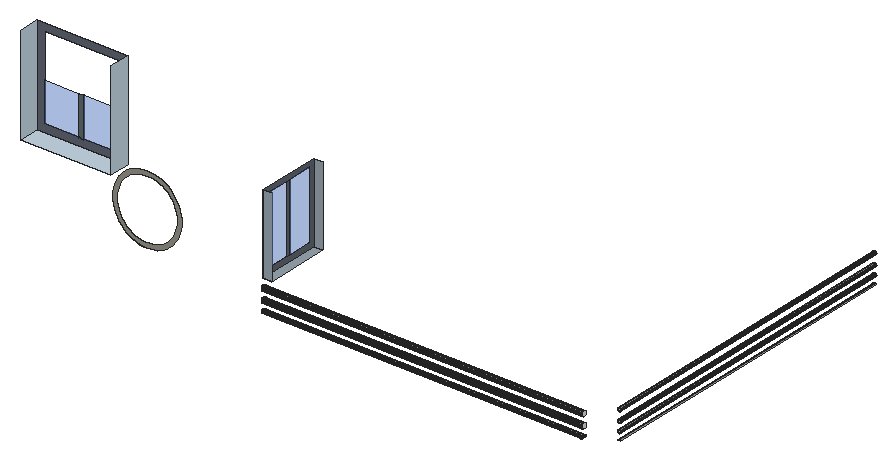
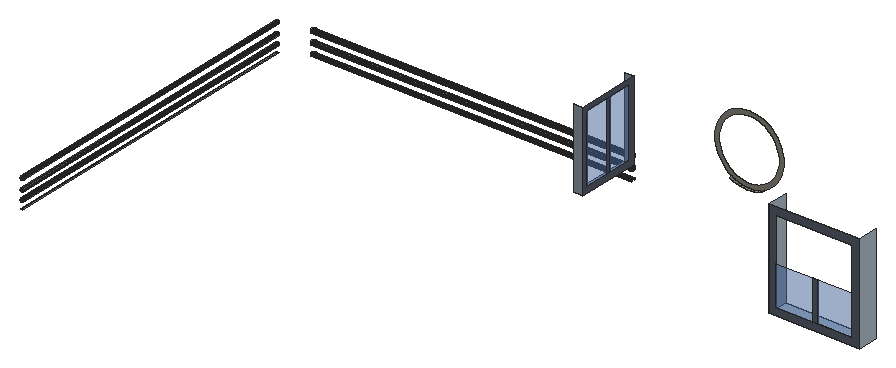
# SketchUp Ruby script. Lengths in inches.
U = 1.inch
M = Sketchup.active_model
def pt(a) = Geom::Point3d.new(a.map { |v| v * U })
def face(e, loops, mat)
  f = e.add_face(loops[0].map { |a| pt(a) })
  loops[1..].each { |l| e.add_face(l.map { |a| pt(a) }).erase! }
  f.material = f.back_material = mat if mat
  f
end
# faces: each face lists its corners as indices into pts; further lists are holes
def faces(e, pts, list, mat = nil) = list.each { |f| face(e, (f[0].is_a?(Array) ? f : [f]).map { |l| l.map { |i| pts[i] } }, mat) }
# xy, xz, yz: faces in a plane at the given z, y or x. An outline is a flat list of corners, or four numbers for a rectangle; further outlines are holes
def ring(l) = l.size == 4 ? [[l[0], l[1]], [l[2], l[1]], [l[2], l[3]], [l[0], l[3]]] : l.each_slice(2).to_a
def flat(e, list, mat, &to3) = list.each { |f| face(e, (f[0].is_a?(Array) ? f : [f]).map { |l| ring(l).map { |u, v| to3.(u, v) } }, mat) }
def xy(e, z, list, mat = nil) = flat(e, list, mat) { |x, y| [x, y, z] }
def xz(e, y, list, mat = nil) = flat(e, list, mat) { |x, z| [x, y, z] }
def yz(e, x, list, mat = nil) = flat(e, list, mat) { |y, z| [x, y, z] }
def lines(e, pts, list) = list.each { |a, b| e.add_line(pt(pts[a]), pt(pts[b])) }
# prism: a flat outline (further loops are holes) pulled along v
def prism(e, loops, v, mat = nil)
  f = face(e, loops, mat); d = Geom::Vector3d.new(v.map { |x| x * U })
  f.pushpull(f.normal.samedirection?(d) ? d.length : -d.length)
end
def box(e, o, s, mat = nil) = prism(e, [[o, [o[0] + s[0], o[1], o[2]], [o[0] + s[0], o[1] + s[1], o[2]], [o[0], o[1] + s[1], o[2]]]], [0, 0, s[2]], mat)
def at(x, y, z, deg = 0) = Geom::Transformation.translation(pt([x, y, z])) * Geom::Transformation.rotation(ORIGIN, Z_AXIS, deg.degrees)
def axes(o, x, y, z) = Geom::Transformation.new([*x, 0, *y, 0, *z, 0, *pt(o).to_a, 1])
def part(name) = M.definitions.add(name)
# library, detail: a bought-in or finely detailed component or shape, given as its bounding box
def library(name, o, s) = part(name).tap { |d| box(d.entities, o, s) }
def detail(e, o, s) = box(e.add_group.entities, o, s)
def put(e, d, t, mat = nil) = e.add_instance(d, t).tap { |i| i.material = mat if mat }
def group(e, t, mat = nil) = e.add_group.tap { |g| g.transformation = t; g.material = mat if mat }.entities
root = M.entities
M.materials.add("[Color M04]").color = [142, 142, 142]
M.materials.add("[Formica Graystone]1").color = [149, 146, 135]
M.materials.add("[Formica Laminate Dark]").color = [95, 101, 114]
M.materials.add("[Formica Speckled Grey]").color = [94, 105, 111]
M.materials.add("[Terrazzo Light Blue]").color = [151, 165, 175]
M.materials.add("[Terrazzo Light Blue]1").color = [196, 214, 227]
M.materials.add("[Translucent Glass Blue]").color = [100, 149, 237]
M.materials["[Translucent Glass Blue]"].alpha = 0.5
xy(root,1990.62,[[605.8,1146.14,928.48,1221.7]],"[Terrazzo Light Blue]1")
xy(root,2047.68,[[1687.83,876.99,1720.33,1103.3]],"[Terrazzo Light Blue]")
xz(root,793.39,[[[1341.18,2057.61,1354.09,2058.29,1366.86,2060.3125,1379.35,2063.66,1391.42,2068.29,1402.93,2074.16,1413.77,2081.2,1423.82,2089.33,1432.96,2098.47,1441.1,2108.52,1448.14,2119.36,1454.01,2130.88,1458.64,2142.95,1461.98,2155.43,1464.01,2168.2,1464.68,2181.11,1464.01,2194.02,1461.98,2206.79,1458.64,2219.28,1454.01,2231.34,1448.14,2242.86,1441.1,2253.7,1432.96,2263.75,1423.82,2272.89,1413.77,2281.03,1402.93,2288.07,1391.42,2293.93,1379.35,2298.57,1366.86,2301.91,1354.09,2303.94,1341.18,2304.61,1328.27,2303.94,1315.51,2301.91,1303.02,2298.57,1290.95,2293.93,1279.43,2288.07,1268.59,2281.03,1258.55,2272.89,1249.4,2263.75,1241.27,2253.7,1234.23,2242.86,1228.36,2231.34,1223.73,2219.28,1220.38,2206.79,1218.36,2194.02,1217.68,2181.11,1218.36,2168.2,1220.38,2155.43,1223.73,2142.95,1228.36,2130.88,1234.23,2119.36,1241.27,2108.52,1249.4,2098.47,1258.55,2089.33,1268.59,2081.2,1279.43,2074.16,1290.95,2068.29,1303.02,2063.66,1315.51,2060.3125,1328.27,2058.29],[1341.18,2073.03,1329.89,2073.62,1318.71,2075.39,1307.78,2078.32,1297.22,2082.37,1287.14,2087.51,1277.65,2093.67,1268.86,2100.79,1260.86,2108.79,1253.74,2117.58,1247.58,2127.07,1242.44,2137.15,1238.39,2147.71,1235.46,2158.64,1233.69,2169.8125,1233.1,2181.11,1233.69,2192.41,1235.46,2203.58,1238.39,2214.51,1242.44,2225.07,1247.58,2235.15,1253.74,2244.64,1260.86,2253.43,1268.86,2261.43,1277.65,2268.55,1287.14,2274.72,1297.22,2279.85,1307.78,2283.91,1318.71,2286.84,1329.89,2288.6,1341.18,2289.2,1352.48,2288.6,1363.66,2286.84,1374.58,2283.91,1385.15,2279.85,1395.23,2274.72,1404.71,2268.55,1413.51,2261.43,1421.51,2253.43,1428.625,2244.64,1434.79,2235.15,1439.92,2225.07,1443.98,2214.51,1446.91,2203.58,1448.68,2192.41,1449.27,2181.11,1448.68,2169.8125,1446.91,2158.64,1443.98,2147.71,1439.92,2137.15,1434.79,2127.07,1428.625,2117.58,1421.51,2108.79,1413.51,2100.79,1404.71,2093.67,1395.23,2087.51,1385.15,2082.37,1374.58,2078.32,1363.66,2075.39,1352.48,2073.62]]],"[Formica Graystone]1")
xz(root,876.99,[[1687.83,2047.68,1720.33,2330.11]],"[Terrazzo Light Blue]")
xz(root,888.17,[[2950.45,1989.28,2952.01,1989.49,2953.45,1990.09,2954.7,1991.04,2955.65,1992.28,2956.25,1993.73,2956.45,1995.28,2956.25,1996.84,2955.65,1998.28,2954.7,1999.53,2953.45,2000.48,2952.01,2001.08,2950.45,2001.28,2948.9,2001.08,2947.45,2000.48,2946.21,1999.53,2945.26,1998.28,2944.66,1996.84,2944.45,1995.28,2944.66,1993.73,2945.26,1992.28,2946.21,1991.04,2947.45,1990.09,2948.9,1989.49],[2950.45,2021.91,2952.01,2022.11,2953.45,2022.71,2954.7,2023.67,2955.65,2024.91,2956.25,2026.36,2956.45,2027.91,2956.25,2029.46,2955.65,2030.91,2954.7,2032.15,2953.45,2033.1,2952.01,2033.7,2950.45,2033.91,2948.9,2033.7,2947.45,2033.1,2946.21,2032.15,2945.26,2030.91,2944.66,2029.46,2944.45,2027.91,2944.66,2026.36,2945.26,2024.91,2946.21,2023.67,2947.45,2022.71,2948.9,2022.11],[2950.45,2059.47,2952.01,2059.68,2953.45,2060.27,2954.7,2061.23,2955.65,2062.47,2956.25,2063.92,2956.45,2065.47,2956.25,2067.02,2955.65,2068.47,2954.7,2069.71,2953.45,2070.67,2952.01,2071.27,2950.45,2071.47,2948.9,2071.27,2947.45,2070.67,2946.21,2069.71,2945.26,2068.47,2944.66,2067.02,2944.45,2065.47,2944.66,2063.92,2945.26,2062.47,2946.21,2061.23,2947.45,2060.27,2948.9,2059.68]])
xz(root,1103.3,[[1687.83,2047.68,1720.33,2330.11]],"[Terrazzo Light Blue]")
xz(root,1221.7,[[[605.8,1990.62,928.48,2340.5],[631.45,2016.28,902.82,2314.84]]],"[Formica Laminate Dark]")
xz(root,1221.7,[[755.72,2016.28,770.95,2158.7]],"[Formica Speckled Grey]")
xz(root,1221.7,[[631.45,2016.28,755.72,2158.7],[770.95,2016.28,902.82,2158.7]],"[Translucent Glass Blue]")
yz(root,605.8,[[1146.14,1990.62,1221.7,2340.5]],"[Terrazzo Light Blue]1")
yz(root,928.48,[[1146.14,1990.62,1221.7,2340.5]],"[Terrazzo Light Blue]1")
yz(root,1687.83,[[[876.99,2047.68,1103.3,2330.11],[896.8,2067.49,1083.49,2310.3]],[981.04,2067.49,994.49,2310.3]],"[Formica Laminate Dark]")
yz(root,1687.83,[[896.8,2067.49,981.04,2310.3],[994.49,2067.49,1083.49,2310.3]],"[Translucent Glass Blue]")
yz(root,2867.16,[[836.16,1998.66,838.2,1998.93,840.1,1999.72,841.73,2000.97,842.98,2002.6,843.77,2004.5,844.04,2006.54,843.77,2008.58,842.98,2010.48,841.73,2012.11,840.1,2013.36,838.2,2014.15,836.16,2014.41,834.125,2014.15,832.22,2013.36,830.59,2012.11,829.34,2010.48,828.55,2008.58,828.29,2006.54,828.55,2004.5,829.34,2002.6,830.59,2000.97,832.22,1999.72,834.125,1998.93],[836.16,2037.54,838.2,2037.81,840.1,2038.59,841.73,2039.85,842.98,2041.48,843.77,2043.375,844.04,2045.41,843.77,2047.45,842.98,2049.35,841.73,2050.98,840.1,2052.23,838.2,2053.02,836.16,2053.29,834.125,2053.02,832.22,2052.23,830.59,2050.98,829.34,2049.35,828.55,2047.45,828.29,2045.41,828.55,2043.375,829.34,2041.48,830.59,2039.85,832.22,2038.59,834.125,2037.81]])
p = [[2946.21,888.17,1967.03],[2947.45,888.17,1967.98],[2947.45,2026.57,1967.98],[2946.21,2026.57,1967.03],[2953.45,888.17,1967.98],[2954.7,888.17,1967.03],
  [2954.7,2026.57,1967.03],[2953.45,2026.57,1967.98],[2867.16,828.55,1967.1875],[2867.16,828.29,1969.23],[1720.33,828.29,1969.23],[1720.33,828.55,1967.1875],
  [2867.16,844.04,1969.23],[2867.16,843.77,1967.1875],[1720.33,843.77,1967.1875],[1720.33,844.04,1969.23],[2948.9,888.17,1968.58],[2948.9,2026.57,1968.58],
  [2952.01,888.17,1968.58],[2952.01,2026.57,1968.58],[2950.45,888.17,1968.78],[2950.45,2026.57,1968.78],[2867.16,828.55,1971.27],[1720.33,828.55,1971.27],
  [2867.16,843.77,1971.27],[1720.33,843.77,1971.27],[2867.16,829.34,1973.16],[1720.33,829.34,1973.16],[2867.16,842.98,1973.16],[1720.33,842.98,1973.16],
  [2867.16,830.59,1974.8],[1720.33,830.59,1974.8],[2867.16,841.73,1974.8],[1720.33,841.73,1974.8],[2867.16,832.22,1976.05],[1720.33,832.22,1976.05],
  [2867.16,840.1,1976.05],[1720.33,840.1,1976.05],[2867.16,834.125,1976.83],[1720.33,834.125,1976.83],[2867.16,838.2,1976.83],[1720.33,838.2,1976.83],
  [2867.16,836.16,1977.1],[1720.33,836.16,1977.1],[2950.45,888.17,1989.28],[2948.9,888.17,1989.49],[2948.9,2026.57,1989.49],[2950.45,2026.57,1989.28],
  [2952.01,888.17,1989.49],[2952.01,2026.57,1989.49],[2947.45,888.17,1990.09],[2947.45,2026.57,1990.09],[2953.45,888.17,1990.09],[2953.45,2026.57,1990.09],
  [2946.21,888.17,1991.04],[2946.21,2026.57,1991.04],[2954.7,888.17,1991.04],[2954.7,2026.57,1991.04],[2945.26,888.17,1992.28],[2945.26,2026.57,1992.28],
  [2955.65,888.17,1992.28],[2955.65,2026.57,1992.28],[2944.66,888.17,1993.73],[2944.66,2026.57,1993.73],[2956.25,888.17,1993.73],[2956.25,2026.57,1993.73],
  [2944.45,888.17,1995.28],[2944.45,2026.57,1995.28],[2956.45,888.17,1995.28],[2956.45,2026.57,1995.28],[2944.66,888.17,1996.84],[2944.66,2026.57,1996.84],
  [2956.25,888.17,1996.84],[2956.25,2026.57,1996.84],[2945.26,888.17,1998.28],[2945.26,2026.57,1998.28],[2955.65,888.17,1998.28],[2955.65,2026.57,1998.28],
  [2946.21,888.17,1999.53],[2946.21,2026.57,1999.53],[2954.7,888.17,1999.53],[2954.7,2026.57,1999.53],[2867.16,836.16,1998.66],[2867.16,834.125,1998.93],
  [1720.33,834.125,1998.93],[1720.33,836.16,1998.66],[2867.16,838.2,1998.93],[1720.33,838.2,1998.93],[2867.16,832.22,1999.72],[1720.33,832.22,1999.72],
  [2867.16,840.1,1999.72],[1720.33,840.1,1999.72],[2947.45,888.17,2000.48],[2947.45,2026.57,2000.48],[2953.45,888.17,2000.48],[2953.45,2026.57,2000.48],
  [2867.16,830.59,2000.97],[1720.33,830.59,2000.97],[2867.16,841.73,2000.97],[1720.33,841.73,2000.97],[2948.9,888.17,2001.08],[2948.9,2026.57,2001.08],
  [2952.01,888.17,2001.08],[2952.01,2026.57,2001.08],[2867.16,829.34,2002.6],[1720.33,829.34,2002.6],[2867.16,842.98,2002.6],[1720.33,842.98,2002.6],
  [2950.45,888.17,2001.28],[2950.45,2026.57,2001.28],[2867.16,828.55,2004.5],[1720.33,828.55,2004.5],[2867.16,843.77,2004.5],[1720.33,843.77,2004.5],
  [2867.16,828.29,2006.54],[1720.33,828.29,2006.54],[2867.16,844.04,2006.54],[1720.33,844.04,2006.54],[2867.16,828.55,2008.58],[1720.33,828.55,2008.58],
  [2867.16,843.77,2008.58],[1720.33,843.77,2008.58],[2867.16,829.34,2010.48],[1720.33,829.34,2010.48],[2867.16,842.98,2010.48],[1720.33,842.98,2010.48],
  [2867.16,830.59,2012.11],[1720.33,830.59,2012.11],[2867.16,841.73,2012.11],[1720.33,841.73,2012.11],[2867.16,832.22,2013.36],[1720.33,832.22,2013.36],
  [2867.16,840.1,2013.36],[1720.33,840.1,2013.36],[2867.16,834.125,2014.15],[1720.33,834.125,2014.15],[2867.16,838.2,2014.15],[1720.33,838.2,2014.15],
  [2867.16,836.16,2014.41],[1720.33,836.16,2014.41],[2950.45,888.17,2021.91],[2948.9,888.17,2022.11],[2948.9,2026.57,2022.11],[2950.45,2026.57,2021.91],
  [2952.01,888.17,2022.11],[2952.01,2026.57,2022.11],[2947.45,888.17,2022.71],[2947.45,2026.57,2022.71],[2953.45,888.17,2022.71],[2953.45,2026.57,2022.71],
  [2946.21,888.17,2023.67],[2946.21,2026.57,2023.67],[2954.7,888.17,2023.67],[2954.7,2026.57,2023.67],[2945.26,888.17,2024.91],[2945.26,2026.57,2024.91],
  [2955.65,888.17,2024.91],[2955.65,2026.57,2024.91],[2944.66,888.17,2026.36],[2944.66,2026.57,2026.36],[2956.25,888.17,2026.36],[2956.25,2026.57,2026.36],
  [2944.45,888.17,2027.91],[2944.45,2026.57,2027.91],[2956.45,888.17,2027.91],[2956.45,2026.57,2027.91],[2944.66,888.17,2029.46],[2944.66,2026.57,2029.46],
  [2956.25,888.17,2029.46],[2956.25,2026.57,2029.46],[2945.26,888.17,2030.91],[2945.26,2026.57,2030.91],[2955.65,888.17,2030.91],[2955.65,2026.57,2030.91],
  [2946.21,888.17,2032.15],[2946.21,2026.57,2032.15],[2954.7,888.17,2032.15],[2954.7,2026.57,2032.15],[2947.45,888.17,2033.1],[2947.45,2026.57,2033.1],
  [2953.45,888.17,2033.1],[2953.45,2026.57,2033.1],[2948.9,888.17,2033.7],[2948.9,2026.57,2033.7],[2952.01,888.17,2033.7],[2952.01,2026.57,2033.7],
  [2950.45,888.17,2033.91],[2950.45,2026.57,2033.91],[2867.16,836.16,2037.54],[2867.16,834.125,2037.81],[1720.33,834.125,2037.81],[1720.33,836.16,2037.54],
  [2867.16,838.2,2037.81],[1720.33,838.2,2037.81],[2867.16,832.22,2038.59],[1720.33,832.22,2038.59],[2867.16,840.1,2038.59],[1720.33,840.1,2038.59],
  [2867.16,830.59,2039.85],[1720.33,830.59,2039.85],[2867.16,841.73,2039.85],[1720.33,841.73,2039.85],[2867.16,829.34,2041.48],[1720.33,829.34,2041.48],
  [2867.16,842.98,2041.48],[1720.33,842.98,2041.48],[2867.16,828.55,2043.375],[1720.33,828.55,2043.375],[2867.16,843.77,2043.375],[1720.33,843.77,2043.375],
  [2867.16,828.29,2045.41],[1720.33,828.29,2045.41],[2867.16,844.04,2045.41],[1720.33,844.04,2045.41],[2867.16,828.55,2047.45],[1720.33,828.55,2047.45],
  [2867.16,843.77,2047.45],[1720.33,843.77,2047.45],[2867.16,829.34,2049.35],[1720.33,829.34,2049.35],[2867.16,842.98,2049.35],[1720.33,842.98,2049.35],
  [2867.16,830.59,2050.98],[1720.33,830.59,2050.98],[2867.16,841.73,2050.98],[1720.33,841.73,2050.98],[2867.16,832.22,2052.23],[1720.33,832.22,2052.23],
  [2867.16,840.1,2052.23],[1720.33,840.1,2052.23],[2867.16,834.125,2053.02],[1720.33,834.125,2053.02],[2867.16,838.2,2053.02],[1720.33,838.2,2053.02],
  [2867.16,836.16,2053.29],[1720.33,836.16,2053.29],[1328.27,803.71,2058.29],[1341.18,803.71,2057.61],[1341.18,793.39,2057.61],[1328.27,793.39,2058.29],
  [1354.09,803.71,2058.29],[1354.09,793.39,2058.29],[1315.51,803.71,2060.3125],[1315.51,793.39,2060.3125],[1366.86,803.71,2060.3125],[1366.86,793.39,2060.3125],
  [2950.45,888.17,2059.47],[2948.9,888.17,2059.68],[2948.9,2026.57,2059.68],[2950.45,2026.57,2059.47],[2952.01,888.17,2059.68],[2952.01,2026.57,2059.68],
  [2947.45,888.17,2060.27],[2947.45,2026.57,2060.27],[2953.45,888.17,2060.27],[2953.45,2026.57,2060.27],[1303.02,803.71,2063.66],[1303.02,793.39,2063.66],
  [1379.35,803.71,2063.66],[1379.35,793.39,2063.66],[2946.21,888.17,2061.23],[2946.21,2026.57,2061.23],[2954.7,888.17,2061.23],[2954.7,2026.57,2061.23],
  [2945.26,888.17,2062.47],[2945.26,2026.57,2062.47],[2955.65,888.17,2062.47],[2955.65,2026.57,2062.47],[2944.66,888.17,2063.92],[2944.66,2026.57,2063.92],
  [2956.25,888.17,2063.92],[2956.25,2026.57,2063.92],[1290.95,803.71,2068.29],[1290.95,793.39,2068.29],[1391.42,803.71,2068.29],[1391.42,793.39,2068.29],
  [2944.45,888.17,2065.47],[2944.45,2026.57,2065.47],[2956.45,888.17,2065.47],[2956.45,2026.57,2065.47],[2944.66,888.17,2067.02],[2944.66,2026.57,2067.02],
  [2956.25,888.17,2067.02],[2956.25,2026.57,2067.02],[2945.26,888.17,2068.47],[2945.26,2026.57,2068.47],[2955.65,888.17,2068.47],[2955.65,2026.57,2068.47],
  [1279.43,803.71,2074.16],[1279.43,793.39,2074.16],[1402.93,803.71,2074.16],[1402.93,793.39,2074.16],[2946.21,888.17,2069.71],[2946.21,2026.57,2069.71],
  [2954.7,888.17,2069.71],[2954.7,2026.57,2069.71],[2947.45,888.17,2070.67],[2947.45,2026.57,2070.67],[2953.45,888.17,2070.67],[2953.45,2026.57,2070.67],
  [2948.9,888.17,2071.27],[2948.9,2026.57,2071.27],[2952.01,888.17,2071.27],[2952.01,2026.57,2071.27],[2950.45,888.17,2071.47],[2950.45,2026.57,2071.47]]
faces(root,p,[[0,1,2,3],[4,5,6,7],[8,9,10,11],[12,13,14,15],[1,16,17,2],[18,4,7,19],[16,20,21,17],[20,18,19,21],
  [9,22,23,10],[24,12,15,25],[22,26,27,23],[28,24,25,29],[26,30,31,27],[32,28,29,33],[30,34,35,31],[36,32,33,37],
  [34,38,39,35],[40,36,37,41],[38,42,43,39],[42,40,41,43],[44,45,46,47],[48,44,47,49],[45,50,51,46],[52,48,49,53],
  [50,54,55,51],[56,52,53,57],[54,58,59,55],[60,56,57,61],[58,62,63,59],[64,60,61,65],[62,66,67,63],[68,64,65,69],
  [66,70,71,67],[72,68,69,73],[70,74,75,71],[76,72,73,77],[74,78,79,75],[80,76,77,81],[82,83,84,85],[86,82,85,87],
  [83,88,89,84],[90,86,87,91],[78,92,93,79],[94,80,81,95],[88,96,97,89],[98,90,91,99],[92,100,101,93],[102,94,95,103],
  [96,104,105,97],[106,98,99,107],[100,108,109,101],[108,102,103,109],[104,110,111,105],[112,106,107,113],[110,114,115,111],[116,112,113,117],
  [114,118,119,115],[120,116,117,121],[118,122,123,119],[124,120,121,125],[122,126,127,123],[128,124,125,129],[126,130,131,127],[132,128,129,133],
  [130,134,135,131],[136,132,133,137],[134,138,139,135],[138,136,137,139],[140,141,142,143],[144,140,143,145],[141,146,147,142],[148,144,145,149],
  [146,150,151,147],[152,148,149,153],[150,154,155,151],[156,152,153,157],[154,158,159,155],[160,156,157,161],[158,162,163,159],[164,160,161,165],
  [162,166,167,163],[168,164,165,169],[166,170,171,167],[172,168,169,173],[170,174,175,171],[176,172,173,177],[174,178,179,175],[180,176,177,181],
  [178,182,183,179],[184,180,181,185],[182,186,187,183],[186,184,185,187],[188,189,190,191],[192,188,191,193],[189,194,195,190],[196,192,193,197],
  [194,198,199,195],[200,196,197,201],[198,202,203,199],[204,200,201,205],[202,206,207,203],[208,204,205,209],[206,210,211,207],[212,208,209,213],
  [210,214,215,211],[216,212,213,217],[214,218,219,215],[220,216,217,221],[218,222,223,219],[224,220,221,225],[222,226,227,223],[228,224,225,229],
  [226,230,231,227],[232,228,229,233],[230,234,235,231],[234,232,233,235],[246,247,248,249],[250,246,249,251],[247,252,253,248],[254,250,251,255],
  [252,260,261,253],[262,254,255,263],[260,264,265,261],[266,262,263,267],[264,268,269,265],[270,266,267,271],[268,276,277,269],[278,270,271,279],
  [276,280,281,277],[282,278,279,283],[280,284,285,281],[286,282,283,287],[284,292,293,285],[294,286,287,295],[292,296,297,293],[298,294,295,299],
  [296,300,301,297],[302,298,299,303],[300,304,305,301],[304,302,303,305]],"[Color M04]")
faces(root,p,[[236,237,238,239],[237,240,241,238],[242,236,239,243],[240,244,245,241],[256,242,243,257],[244,258,259,245],[272,256,257,273],[258,274,275,259],
  [288,272,273,289],[274,290,291,275]],"[Formica Graystone]1")
